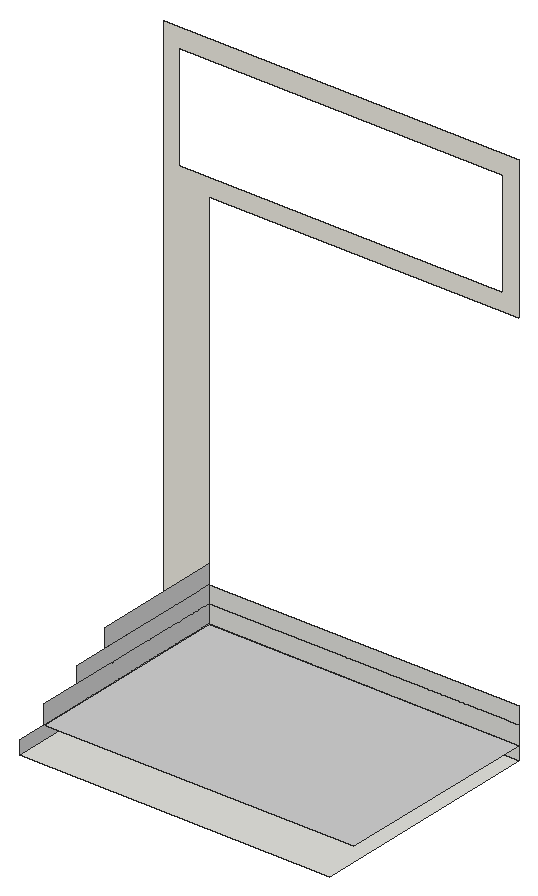
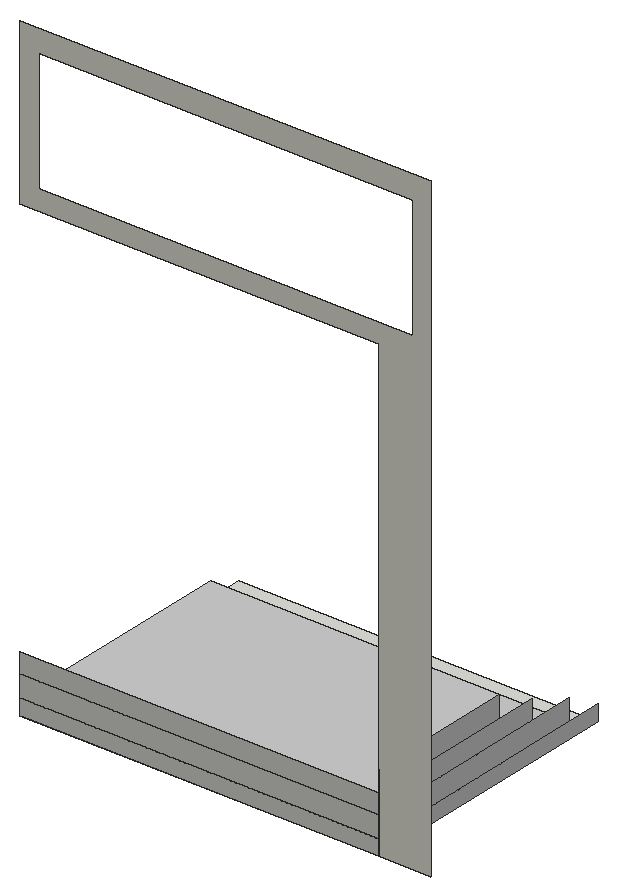
# SketchUp Ruby script. Lengths in inches.
U = 1.inch
M = Sketchup.active_model
def pt(a) = Geom::Point3d.new(a.map { |v| v * U })
def face(e, loops, mat)
  f = e.add_face(loops[0].map { |a| pt(a) })
  loops[1..].each { |l| e.add_face(l.map { |a| pt(a) }).erase! }
  f.material = f.back_material = mat if mat
  f
end
# faces: each face lists its corners as indices into pts; further lists are holes
def faces(e, pts, list, mat = nil) = list.each { |f| face(e, (f[0].is_a?(Array) ? f : [f]).map { |l| l.map { |i| pts[i] } }, mat) }
# xy, xz, yz: faces in a plane at the given z, y or x. An outline is a flat list of corners, or four numbers for a rectangle; further outlines are holes
def ring(l) = l.size == 4 ? [[l[0], l[1]], [l[2], l[1]], [l[2], l[3]], [l[0], l[3]]] : l.each_slice(2).to_a
def flat(e, list, mat, &to3) = list.each { |f| face(e, (f[0].is_a?(Array) ? f : [f]).map { |l| ring(l).map { |u, v| to3.(u, v) } }, mat) }
def xy(e, z, list, mat = nil) = flat(e, list, mat) { |x, y| [x, y, z] }
def xz(e, y, list, mat = nil) = flat(e, list, mat) { |x, z| [x, y, z] }
def yz(e, x, list, mat = nil) = flat(e, list, mat) { |y, z| [x, y, z] }
def lines(e, pts, list) = list.each { |a, b| e.add_line(pt(pts[a]), pt(pts[b])) }
# prism: a flat outline (further loops are holes) pulled along v
def prism(e, loops, v, mat = nil)
  f = face(e, loops, mat); d = Geom::Vector3d.new(v.map { |x| x * U })
  f.pushpull(f.normal.samedirection?(d) ? d.length : -d.length)
end
def box(e, o, s, mat = nil) = prism(e, [[o, [o[0] + s[0], o[1], o[2]], [o[0] + s[0], o[1] + s[1], o[2]], [o[0], o[1] + s[1], o[2]]]], [0, 0, s[2]], mat)
def at(x, y, z, deg = 0) = Geom::Transformation.translation(pt([x, y, z])) * Geom::Transformation.rotation(ORIGIN, Z_AXIS, deg.degrees)
def axes(o, x, y, z) = Geom::Transformation.new([*x, 0, *y, 0, *z, 0, *pt(o).to_a, 1])
def part(name) = M.definitions.add(name)
# library, detail: a bought-in or finely detailed component or shape, given as its bounding box
def library(name, o, s) = part(name).tap { |d| box(d.entities, o, s) }
def detail(e, o, s) = box(e.add_group.entities, o, s)
def put(e, d, t, mat = nil) = e.add_instance(d, t).tap { |i| i.material = mat if mat }
def group(e, t, mat = nil) = e.add_group.tap { |g| g.transformation = t; g.material = mat if mat }.entities
root = M.entities
M.materials.add("[Carrera Marble]").color = [207, 207, 207]
M.materials.add("[Tile Limestone Large]").color = [237, 234, 224]
xy(root,17.625,[[111.93,47.98,355.29,233.86]])
xy(root,28.22,[[111.93,71.98,355.29,233.86]],"[Carrera Marble]")
xz(root,233.86,[[111.93,17.625,355.29,28.22],[111.93,28.22,355.29,42.68],[111.93,42.68,355.29,56.07]])
xz(root,233.86,[[[76.4,17.625,111.93,17.625,111.93,328.93,355.29,328.93,355.29,440.5625,76.4,440.5625],[88.43,342.19,342.93,425.32]]],"[Tile Limestone Large]")
yz(root,111.93,[[47.98,17.625,233.86,28.22],[71.98,28.22,233.86,42.68],[103.86,42.68,233.86,56.07],[131.48,56.07,233.86,70.61]],"[Carrera Marble]")
